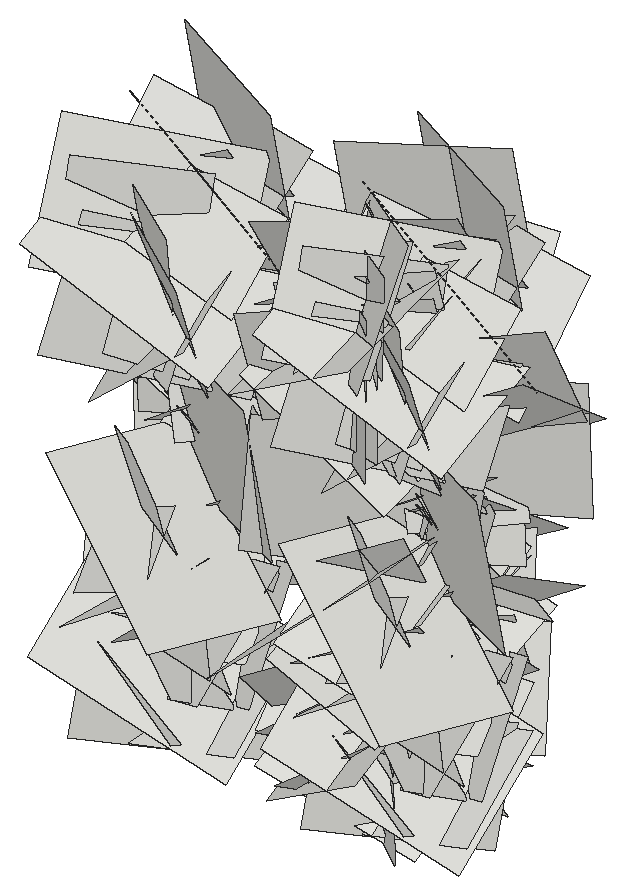
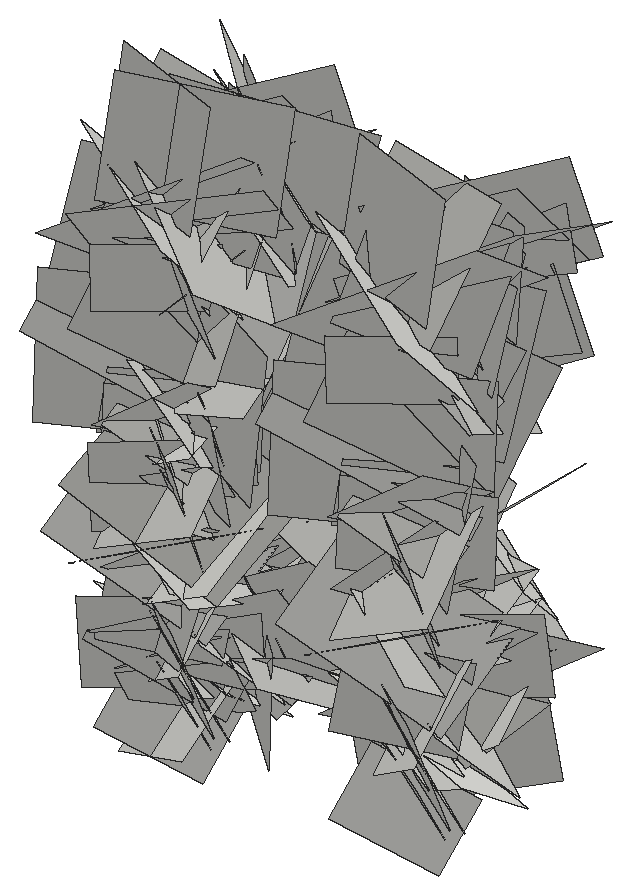
# SketchUp Ruby script. Lengths in inches.
U = 1.inch
M = Sketchup.active_model
def pt(a) = Geom::Point3d.new(a.map { |v| v * U })
def face(e, loops, mat)
  f = e.add_face(loops[0].map { |a| pt(a) })
  loops[1..].each { |l| e.add_face(l.map { |a| pt(a) }).erase! }
  f.material = f.back_material = mat if mat
  f
end
# faces: each face lists its corners as indices into pts; further lists are holes
def faces(e, pts, list, mat = nil) = list.each { |f| face(e, (f[0].is_a?(Array) ? f : [f]).map { |l| l.map { |i| pts[i] } }, mat) }
# xy, xz, yz: faces in a plane at the given z, y or x. An outline is a flat list of corners, or four numbers for a rectangle; further outlines are holes
def ring(l) = l.size == 4 ? [[l[0], l[1]], [l[2], l[1]], [l[2], l[3]], [l[0], l[3]]] : l.each_slice(2).to_a
def flat(e, list, mat, &to3) = list.each { |f| face(e, (f[0].is_a?(Array) ? f : [f]).map { |l| ring(l).map { |u, v| to3.(u, v) } }, mat) }
def xy(e, z, list, mat = nil) = flat(e, list, mat) { |x, y| [x, y, z] }
def xz(e, y, list, mat = nil) = flat(e, list, mat) { |x, z| [x, y, z] }
def yz(e, x, list, mat = nil) = flat(e, list, mat) { |y, z| [x, y, z] }
def lines(e, pts, list) = list.each { |a, b| e.add_line(pt(pts[a]), pt(pts[b])) }
# prism: a flat outline (further loops are holes) pulled along v
def prism(e, loops, v, mat = nil)
  f = face(e, loops, mat); d = Geom::Vector3d.new(v.map { |x| x * U })
  f.pushpull(f.normal.samedirection?(d) ? d.length : -d.length)
end
def box(e, o, s, mat = nil) = prism(e, [[o, [o[0] + s[0], o[1], o[2]], [o[0] + s[0], o[1] + s[1], o[2]], [o[0], o[1] + s[1], o[2]]]], [0, 0, s[2]], mat)
def at(x, y, z, deg = 0) = Geom::Transformation.translation(pt([x, y, z])) * Geom::Transformation.rotation(ORIGIN, Z_AXIS, deg.degrees)
def axes(o, x, y, z) = Geom::Transformation.new([*x, 0, *y, 0, *z, 0, *pt(o).to_a, 1])
def part(name) = M.definitions.add(name)
# library, detail: a bought-in or finely detailed component or shape, given as its bounding box
def library(name, o, s) = part(name).tap { |d| box(d.entities, o, s) }
def detail(e, o, s) = box(e.add_group.entities, o, s)
def put(e, d, t, mat = nil) = e.add_instance(d, t).tap { |i| i.material = mat if mat }
def group(e, t, mat = nil) = e.add_group.tap { |g| g.transformation = t; g.material = mat if mat }.entities
root = M.entities
c1 = part("Component\#6")
p = [[0.01,0,0],[0,3.24,4.54],[4.32,3.24,4.54],[4.33,0,0]]
faces(c1.entities,p,[[0,1,2,3]])
put(root,c1,axes([28.31,207.72,1.15],[0.00392,-0.70388,0.63123],[0.16138,0.62344,0.69431],[-0.98911,0.09893,0.11578]))
put(root,c1,axes([28.31,208.64,6.82],[-0.0498,0.28937,-0.67344],[-0.06797,-0.67386,-0.28508],[-0.77398,0.04056,0.06836]))
put(root,c1,axes([24.34,203.75,8.58],[0.14047,0.70659,0.15459],[-0.00867,0.15861,-0.71798],[0.76665,-0.12767,-0.03644]))
put(root,c1,axes([24.34,201.6875,18.6875],[0.06388,0.10125,0.82658],[-0.05301,0.82768,-0.09774],[0.88113,0.04245,-0.0658]))
put(root,c1,axes([24.34,204.41,7.91],[0.10208,-0.52254,-0.48763],[0.08086,-0.48171,0.53127],[0.75328,0.12252,0.00905]))
put(root,c1,axes([24.34,205.98,8.7],[-0.1184,0.10295,0.88925],[0.12891,0.88959,-0.08771],[0.94011,-0.10902,0.12403]))
put(root,c1,axes([28.31,205.95,7.64],[0.13368,0.21915,0.90835],[0.05222,0.91375,-0.2273],[-0.9891,0.07786,0.11076]))
put(root,c1,axes([28.31,207.38,2.3],[-0.03327,0.56132,-0.40527],[-0.08729,-0.40584,-0.55572],[-0.72866,0.02299,0.08508]))
put(root,c1,axes([24.34,210.56,5.71],[-0.17873,-0.295,-0.9769],[0.02803,-0.99107,0.29472],[1.08133,-0.02307,-0.16911]))
put(root,c1,axes([24.34,206,12.43],[0.16769,0.64159,0.3622],[-0.01184,0.3725,-0.65496],[0.78088,-0.13213,-0.08771]))
put(root,c1,axes([24.34,202.81,3.34],[-0.17899,0.36268,0.93898],[0.06935,0.95405,-0.35673],[1.06473,-0.00117,0.18108]))
put(root,c1,axes([24.34,204.45,21.63],[-0.07523,0.18922,-0.91056],[0.04715,-0.91147,-0.19287],[0.98469,0.0581,-0.06033]))
put(root,c1,axes([28.31,205.65,3.3125],[-0.06993,0.62057,0.27964],[-0.0119,0.27992,-0.62384],[-0.72141,-0.06477,-0.01682]))
put(root,c1,axes([24.34,207.17,17.14],[0.0563,-0.55845,0.63654],[0.00808,0.63808,0.55916],[0.89756,0.02928,-0.04497]))
put(root,c1,axes([28.31,206.6,8.35],[-0.07615,0.29672,0.54367],[-0.07213,0.54022,-0.30383],[-0.65256,-0.09434,-0.02986]))
put(root,c1,axes([28.31,204.05,18.57],[-0.06151,0.80519,-0.14469],[0.18353,-0.12968,-0.7911],[-0.84753,-0.08652,-0.16081]))
put(root,c1,axes([28.31,206.67,12.85],[-0.04142,0.63331,-0.27554],[-0.00251,-0.27611,-0.63426],[-0.73209,-0.03488,0.01776]))
put(root,c1,axes([24.34,205.78,7.5],[-0.02909,0.83454,0.28231],[0.13137,0.2833,-0.8254],[0.92457,-0.01399,0.12617]))
put(root,c1,axes([28.31,206.02,7.14],[-0.00935,0.6115,0.38278],[0.02819,0.38283,-0.61096],[-0.76419,0.00664,-0.02722]))
put(root,c1,axes([28.31,206.15,0.87],[0.01906,0.33732,0.58365],[-0.0637,0.58234,-0.33471],[-0.71172,-0.04309,0.04558]))
put(root,c1,axes([24.34,206.11,11.76],[-0.09648,-0.72051,0.9522],[-0.19874,0.95174,0.70224],[1.25002,0.0957,0.18514]))
put(root,c1,axes([28.31,205.78,22.17],[-0.00372,0.37911,-0.54343],[-0.01311,-0.54338,-0.37899],[-0.70223,0.00813,0.00995]))
put(root,c1,axes([24.34,201.43,15.61],[0.13511,0.17275,0.7909],[0.07376,0.79534,-0.18493],[0.85494,-0.09592,-0.10904]))
put(root,c1,axes([28.31,205.06,0.06],[0.16762,-0.72435,0.3647],[0.00744,0.37278,0.73735],[-0.85961,-0.13802,0.0775]))
put(root,c1,axes([28.31,203.18,8],[-0.06036,-0.35202,0.5516],[0.07606,0.54699,0.35648],[-0.68943,0.09116,-0.00896]))
put(root,c1,axes([24.34,200.34,18.7],[-0.08817,0.51183,1.11442],[-0.20058,1.09825,-0.51853],[1.28435,0.20665,-0.00447]))
put(root,c1,axes([28.31,200.61,7.25],[0.15258,0.77944,0.1154],[0.02035,0.1138,-0.79262],[-0.83497,0.14521,0.00177]))
put(root,c1,axes([28.31,209.54,8.98],[-0.01886,-0.65319,-0.4186],[0.2021,-0.40955,0.63097],[-0.79714,-0.08839,0.16987]))
put(root,c1,axes([28.31,205.68,16.84],[-0.07036,-0.63328,-0.02287],[0.09357,-0.03201,0.6302],[-0.66517,0.06248,0.09107]))
put(root,c1,axes([24.34,211.08,20.1875],[-0.1855,-0.74932,-0.85781],[0.09412,-0.87421,0.74553],[1.20366,-0.04712,-0.19049]))
put(root,c1,axes([24.34,206.49,12.28],[-0.17995,0.92169,-0.62911],[0.1265,-0.6177,-0.93718],[1.17609,0.20746,0.00455]))
put(root,c1,axes([28.31,209.83,18.53],[0.13516,-0.18826,-0.70807],[0.00477,-0.7185,0.19184],[-0.77662,-0.03718,-0.12206]))
put(root,c1,axes([28.31,203.04,6.2],[0.19197,0.78573,-0.28472],[0.09491,-0.3079,-0.79273],[-0.88077,0.13807,-0.14748]))
put(root,c1,axes([28.31,202.62,14.39],[0.09007,0.1944,0.61889],[-0.03503,0.62466,-0.19168],[-0.68673,-0.00637,0.09095]))
put(root,c1,axes([24.34,203.52,7.375],[0.0121,1.00291,-0.55649],[-0.12117,-0.55275,-0.99852],[1.20972,-0.0654,-0.09445]))
put(root,c1,axes([24.34,203.17,19.17],[-0.16233,1.06667,0.75788],[-0.09967,0.75211,-1.07754],[1.38342,0.17935,0.0113]))
put(root,c1,axes([24.34,202.39,0.06],[0.12593,0.12266,1.10922],[-0.15067,1.10807,-0.10731],[1.17331,0.12913,-0.13284]))
put(root,c1,axes([24.34,208.78,4.43],[0.01106,-0.99025,0.53374],[0.00744,0.53381,0.99025],[1.19241,0.00586,-0.01113]))
put(root,c1,axes([24.34,208.53,24.44],[0.00063,0.23668,-1.01361],[0.18606,-0.99912,-0.23319],[1.08753,0.17079,0.04049]))
put(root,c1,axes([24.34,200.25,4.04],[-0.10038,1.14624,0.70824],[-0.13093,0.69961,-1.1488],[1.42222,0.14531,-0.05578]))
put(root,c1,axes([24.34,209.01,4.56],[-0.09462,-0.88739,-0.86898],[0.02241,-0.87218,0.88849],[1.31634,-0.04894,-0.07759]))
put(root,c1,axes([28.31,208.89,13.53],[0.18208,-0.09561,-0.67164],[0.05748,-0.68868,0.1119],[-0.71681,-0.07951,-0.16163]))
put(root,c1,axes([24.34,207.09,15.04],[0.15807,-1.02909,-0.4958],[-0.14338,-0.5124,1.02286],[1.20232,0.07419,0.18716]))
put(root,c1,axes([24.34,204.39,20.61],[0.01972,0.37325,-1.09096],[0.03348,-1.09086,-0.37268],[1.22177,0.02387,0.02782]))
put(root,c1,axes([24.34,203.64,8.5],[0.20575,0.76434,-0.74551],[-0.06488,-0.74852,-0.78336],[1.12991,-0.18216,0.09078]))
put(root,c1,axes([24.34,209.96,4.13],[0.07876,-0.66244,-0.94852],[0.03994,-0.94858,0.66543],[1.2257,0.07348,0.03927]))
put(root,c1,axes([24.34,199.86,19.8],[-0.08167,1.25653,0.46028],[0.00634,0.46136,-1.25848],[1.41846,0.07029,0.03212]))
put(root,c1,axes([24.34,200.79,15.19],[0.21334,0.28139,1.2169],[-0.22593,1.22225,-0.24738],[1.30453,0.16566,-0.24185]))
put(root,c1,axes([24.34,201.07,18.92],[0.13602,0.69446,0.8684],[0.06726,0.86816,-0.70365],[1.17673,-0.1299,-0.06016]))
put(root,c1,axes([24.34,207.71,2.15],[0.07423,-0.90085,-0.6111],[0.34403,-0.56723,0.87337],[1.1014,0.23789,-0.23162]))
put(root,c1,axes([24.34,206.09,10.75],[0.05447,-0.13377,1.26127],[0.13355,1.2566,0.12815],[1.33779,-0.12,-0.06414]))
put(root,c1,axes([24.34,201.2,11.35],[0.2643,1.29708,-0.17492],[-0.19217,-0.14212,-1.31229],[1.37397,-0.26938,-0.1499]))
put(root,c1,axes([24.34,207.28,11.15],[0.07738,-1.09853,0.81062],[0.01823,0.81245,1.09947],[1.44703,0.04851,-0.0572]))
put(root,c1,axes([24.34,205.65,23.04],[0.12198,0.70336,-1.01008],[0.22842,-1.01033,-0.67899],[1.28455,0.11286,0.21665]))
put(root,c1,axes([24.34,205.49,13.28],[0.13832,-0.68419,1.12815],[0.08396,1.13567,0.67959],[1.39605,-0.00051,-0.15265]))
put(root,c1,axes([24.34,206.9375,13.83],[0.19711,0.10382,-1.30915],[0.13395,-1.31749,-0.08653],[1.38559,0.11259,0.1946]))
put(root,c1,axes([38.11,206.9375,13.83],[-0.19711,0.10382,-1.30915],[-0.13395,-1.31749,-0.08653],[-1.38559,0.11259,0.1946]))
put(root,c1,axes([38.11,205.49,13.28],[-0.13832,-0.68419,1.12815],[-0.08396,1.13567,0.67959],[-1.39605,-0.00051,-0.15265]))
put(root,c1,axes([38.11,205.65,23.04],[-0.12198,0.70336,-1.01008],[-0.22842,-1.01033,-0.67899],[-1.28455,0.11286,0.21665]))
put(root,c1,axes([38.11,207.28,11.15],[-0.07738,-1.09853,0.81062],[-0.01823,0.81245,1.09947],[-1.44703,0.04851,-0.0572]))
put(root,c1,axes([38.11,201.2,11.35],[-0.2643,1.29708,-0.17492],[0.19217,-0.14212,-1.31229],[-1.37397,-0.26938,-0.1499]))
put(root,c1,axes([38.11,206.09,10.75],[-0.05447,-0.13377,1.26127],[-0.13355,1.2566,0.12815],[-1.33779,-0.12,-0.06414]))
put(root,c1,axes([38.11,207.71,2.15],[-0.07423,-0.90085,-0.6111],[-0.34403,-0.56723,0.87337],[-1.1014,0.23789,-0.23162]))
put(root,c1,axes([38.11,201.07,18.92],[-0.13602,0.69446,0.8684],[-0.06726,0.86816,-0.70365],[-1.17673,-0.1299,-0.06016]))
put(root,c1,axes([38.11,200.79,15.19],[-0.21334,0.28139,1.2169],[0.22593,1.22225,-0.24738],[-1.30453,0.16566,-0.24185]))
put(root,c1,axes([38.11,199.86,19.8],[0.08167,1.25653,0.46028],[-0.00634,0.46136,-1.25848],[-1.41846,0.07029,0.03212]))
put(root,c1,axes([38.11,209.96,4.13],[-0.07876,-0.66244,-0.94852],[-0.03994,-0.94858,0.66543],[-1.2257,0.07348,0.03927]))
put(root,c1,axes([38.11,203.64,8.5],[-0.20575,0.76434,-0.74551],[0.06488,-0.74852,-0.78336],[-1.12991,-0.18216,0.09078]))
put(root,c1,axes([38.11,204.39,20.61],[-0.01972,0.37325,-1.09096],[-0.03348,-1.09086,-0.37268],[-1.22177,0.02387,0.02782]))
put(root,c1,axes([38.11,207.09,15.04],[-0.15807,-1.02909,-0.4958],[0.14338,-0.5124,1.02286],[-1.20232,0.07419,0.18716]))
put(root,c1,axes([34.14,208.89,13.53],[-0.18208,-0.09561,-0.67164],[-0.05748,-0.68868,0.1119],[0.71681,-0.07951,-0.16163]))
put(root,c1,axes([38.11,209.01,4.56],[0.09462,-0.88739,-0.86898],[-0.02241,-0.87218,0.88849],[-1.31634,-0.04894,-0.07759]))
put(root,c1,axes([38.11,200.25,4.04],[0.10038,1.14624,0.70824],[0.13093,0.69961,-1.1488],[-1.42222,0.14531,-0.05578]))
put(root,c1,axes([38.11,208.53,24.44],[-0.00063,0.23668,-1.01361],[-0.18606,-0.99912,-0.23319],[-1.08753,0.17079,0.04049]))
put(root,c1,axes([38.11,208.78,4.43],[-0.01106,-0.99025,0.53374],[-0.00744,0.53381,0.99025],[-1.19241,0.00586,-0.01113]))
put(root,c1,axes([38.11,202.39,0.06],[-0.12593,0.12266,1.10922],[0.15067,1.10807,-0.10731],[-1.17331,0.12913,-0.13284]))
put(root,c1,axes([38.11,203.17,19.17],[0.16233,1.06667,0.75788],[0.09967,0.75211,-1.07754],[-1.38342,0.17935,0.0113]))
put(root,c1,axes([38.11,203.52,7.375],[-0.0121,1.00291,-0.55649],[0.12117,-0.55275,-0.99852],[-1.20972,-0.0654,-0.09445]))
put(root,c1,axes([34.14,202.62,14.39],[-0.09007,0.1944,0.61889],[0.03503,0.62466,-0.19168],[0.68673,-0.00637,0.09095]))
put(root,c1,axes([34.14,203.04,6.2],[-0.19197,0.78573,-0.28472],[-0.09491,-0.3079,-0.79273],[0.88077,0.13807,-0.14748]))
put(root,c1,axes([34.14,209.83,18.53],[-0.13516,-0.18826,-0.70807],[-0.00477,-0.7185,0.19184],[0.77662,-0.03718,-0.12206]))
put(root,c1,axes([38.11,206.49,12.28],[0.17995,0.92169,-0.62911],[-0.1265,-0.6177,-0.93718],[-1.17609,0.20746,0.00455]))
put(root,c1,axes([38.11,211.08,20.1875],[0.1855,-0.74932,-0.85781],[-0.09412,-0.87421,0.74553],[-1.20366,-0.04712,-0.19049]))
put(root,c1,axes([34.14,205.68,16.84],[0.07036,-0.63328,-0.02287],[-0.09357,-0.03201,0.6302],[0.66517,0.06248,0.09107]))
put(root,c1,axes([34.14,209.54,8.98],[0.01886,-0.65319,-0.4186],[-0.2021,-0.40955,0.63097],[0.79714,-0.08839,0.16987]))
put(root,c1,axes([34.14,200.61,7.25],[-0.15258,0.77944,0.1154],[-0.02035,0.1138,-0.79262],[0.83497,0.14521,0.00177]))
put(root,c1,axes([38.11,200.34,18.7],[0.08817,0.51183,1.11442],[0.20058,1.09825,-0.51853],[-1.28435,0.20665,-0.00447]))
put(root,c1,axes([34.14,203.18,8],[0.06036,-0.35202,0.5516],[-0.07606,0.54699,0.35648],[0.68943,0.09116,-0.00896]))
put(root,c1,axes([34.14,205.06,0.06],[-0.16762,-0.72435,0.3647],[-0.00744,0.37278,0.73735],[0.85961,-0.13802,0.0775]))
put(root,c1,axes([38.11,201.43,15.61],[-0.13511,0.17275,0.7909],[-0.07376,0.79534,-0.18493],[-0.85494,-0.09592,-0.10904]))
put(root,c1,axes([34.14,205.78,22.17],[0.00372,0.37911,-0.54343],[0.01311,-0.54338,-0.37899],[0.70223,0.00813,0.00995]))
put(root,c1,axes([38.11,206.11,11.76],[0.09648,-0.72051,0.9522],[0.19874,0.95174,0.70224],[-1.25002,0.0957,0.18514]))
put(root,c1,axes([34.14,206.15,0.87],[-0.01906,0.33732,0.58365],[0.0637,0.58234,-0.33471],[0.71172,-0.04309,0.04558]))
put(root,c1,axes([34.14,206.02,7.14],[0.00935,0.6115,0.38278],[-0.02819,0.38283,-0.61096],[0.76419,0.00664,-0.02722]))
put(root,c1,axes([38.11,205.78,7.5],[0.02909,0.83454,0.28231],[-0.13137,0.2833,-0.8254],[-0.92457,-0.01399,0.12617]))
put(root,c1,axes([34.14,206.67,12.85],[0.04142,0.63331,-0.27554],[0.00251,-0.27611,-0.63426],[0.73209,-0.03488,0.01776]))
put(root,c1,axes([34.14,204.05,18.57],[0.06151,0.80519,-0.14469],[-0.18353,-0.12968,-0.7911],[0.84753,-0.08652,-0.16081]))
put(root,c1,axes([34.14,206.6,8.35],[0.07615,0.29672,0.54367],[0.07213,0.54022,-0.30383],[0.65256,-0.09434,-0.02986]))
put(root,c1,axes([38.11,207.17,17.14],[-0.0563,-0.55845,0.63654],[-0.00808,0.63808,0.55916],[-0.89756,0.02928,-0.04497]))
put(root,c1,axes([34.14,205.65,3.3125],[0.06993,0.62057,0.27964],[0.0119,0.27992,-0.62384],[0.72141,-0.06477,-0.01682]))
put(root,c1,axes([38.11,204.45,21.63],[0.07523,0.18922,-0.91056],[-0.04715,-0.91147,-0.19287],[-0.98469,0.0581,-0.06033]))
put(root,c1,axes([38.11,202.81,3.34],[0.17899,0.36268,0.93898],[-0.06935,0.95405,-0.35673],[-1.06473,-0.00117,0.18108]))
put(root,c1,axes([38.11,206,12.43],[-0.16769,0.64159,0.3622],[0.01184,0.3725,-0.65496],[-0.78088,-0.13213,-0.08771]))
put(root,c1,axes([38.11,210.56,5.71],[0.17873,-0.295,-0.9769],[-0.02803,-0.99107,0.29472],[-1.08133,-0.02307,-0.16911]))
put(root,c1,axes([34.14,207.38,2.3],[0.03327,0.56132,-0.40527],[0.08729,-0.40584,-0.55572],[0.72866,0.02299,0.08508]))
put(root,c1,axes([34.14,205.95,7.64],[-0.13368,0.21915,0.90835],[-0.05222,0.91375,-0.2273],[0.9891,0.07786,0.11076]))
put(root,c1,axes([38.11,205.98,8.7],[0.1184,0.10295,0.88925],[-0.12891,0.88959,-0.08771],[-0.94011,-0.10902,0.12403]))
put(root,c1,axes([38.11,204.41,7.91],[-0.10208,-0.52254,-0.48763],[-0.08086,-0.48171,0.53127],[-0.75328,0.12252,0.00905]))
put(root,c1,axes([38.11,201.6875,18.6875],[-0.06388,0.10125,0.82658],[0.05301,0.82768,-0.09774],[-0.88113,0.04245,-0.0658]))
put(root,c1,axes([38.11,203.75,8.58],[-0.14047,0.70659,0.15459],[0.00867,0.15861,-0.71798],[-0.76665,-0.12767,-0.03644]))
put(root,c1,axes([34.14,208.64,6.82],[0.0498,0.28937,-0.67344],[0.06797,-0.67386,-0.28508],[0.77398,0.04056,0.06836]))
put(root,c1,axes([34.14,207.72,1.15],[-0.00392,-0.70388,0.63123],[-0.16138,0.62344,0.69431],[0.98911,0.09893,0.11578]))
put(root,c1,axes([38.11,207.72,1.15],[0.00392,-0.70388,0.63123],[0.16138,0.62344,0.69431],[-0.98911,0.09893,0.11578]))
put(root,c1,axes([38.11,208.64,6.82],[-0.0498,0.28937,-0.67344],[-0.06797,-0.67386,-0.28508],[-0.77398,0.04056,0.06836]))
put(root,c1,axes([34.14,203.75,8.58],[0.14047,0.70659,0.15459],[-0.00867,0.15861,-0.71798],[0.76665,-0.12767,-0.03644]))
put(root,c1,axes([34.14,201.6875,18.6875],[0.06388,0.10125,0.82658],[-0.05301,0.82768,-0.09774],[0.88113,0.04245,-0.0658]))
put(root,c1,axes([34.14,204.41,7.91],[0.10208,-0.52254,-0.48763],[0.08086,-0.48171,0.53127],[0.75328,0.12252,0.00905]))
put(root,c1,axes([34.14,205.98,8.7],[-0.1184,0.10295,0.88925],[0.12891,0.88959,-0.08771],[0.94011,-0.10902,0.12403]))
put(root,c1,axes([38.11,205.95,7.64],[0.13368,0.21915,0.90835],[0.05222,0.91375,-0.2273],[-0.9891,0.07786,0.11076]))
put(root,c1,axes([38.11,207.38,2.3],[-0.03327,0.56132,-0.40527],[-0.08729,-0.40584,-0.55572],[-0.72866,0.02299,0.08508]))
put(root,c1,axes([34.14,210.56,5.71],[-0.17873,-0.295,-0.9769],[0.02803,-0.99107,0.29472],[1.08133,-0.02307,-0.16911]))
put(root,c1,axes([34.14,206,12.43],[0.16769,0.64159,0.3622],[-0.01184,0.3725,-0.65496],[0.78088,-0.13213,-0.08771]))
put(root,c1,axes([34.14,202.81,3.34],[-0.17899,0.36268,0.93898],[0.06935,0.95405,-0.35673],[1.06473,-0.00117,0.18108]))
put(root,c1,axes([34.14,204.45,21.63],[-0.07523,0.18922,-0.91056],[0.04715,-0.91147,-0.19287],[0.98469,0.0581,-0.06033]))
put(root,c1,axes([38.11,205.65,3.3125],[-0.06993,0.62057,0.27964],[-0.0119,0.27992,-0.62384],[-0.72141,-0.06477,-0.01682]))
put(root,c1,axes([34.14,207.17,17.14],[0.0563,-0.55845,0.63654],[0.00808,0.63808,0.55916],[0.89756,0.02928,-0.04497]))
put(root,c1,axes([38.11,206.6,8.35],[-0.07615,0.29672,0.54367],[-0.07213,0.54022,-0.30383],[-0.65256,-0.09434,-0.02986]))
put(root,c1,axes([38.11,204.05,18.57],[-0.06151,0.80519,-0.14469],[0.18353,-0.12968,-0.7911],[-0.84753,-0.08652,-0.16081]))
put(root,c1,axes([38.11,206.67,12.85],[-0.04142,0.63331,-0.27554],[-0.00251,-0.27611,-0.63426],[-0.73209,-0.03488,0.01776]))
put(root,c1,axes([34.14,205.78,7.5],[-0.02909,0.83454,0.28231],[0.13137,0.2833,-0.8254],[0.92457,-0.01399,0.12617]))
put(root,c1,axes([38.11,206.02,7.14],[-0.00935,0.6115,0.38278],[0.02819,0.38283,-0.61096],[-0.76419,0.00664,-0.02722]))
put(root,c1,axes([38.11,206.15,0.87],[0.01906,0.33732,0.58365],[-0.0637,0.58234,-0.33471],[-0.71172,-0.04309,0.04558]))
put(root,c1,axes([34.14,206.11,11.76],[-0.09648,-0.72051,0.9522],[-0.19874,0.95174,0.70224],[1.25002,0.0957,0.18514]))
put(root,c1,axes([38.11,205.78,22.17],[-0.00372,0.37911,-0.54343],[-0.01311,-0.54338,-0.37899],[-0.70223,0.00813,0.00995]))
put(root,c1,axes([34.14,201.43,15.61],[0.13511,0.17275,0.7909],[0.07376,0.79534,-0.18493],[0.85494,-0.09592,-0.10904]))
put(root,c1,axes([38.11,205.06,0.06],[0.16762,-0.72435,0.3647],[0.00744,0.37278,0.73735],[-0.85961,-0.13802,0.0775]))
put(root,c1,axes([38.11,203.18,8],[-0.06036,-0.35202,0.5516],[0.07606,0.54699,0.35648],[-0.68943,0.09116,-0.00896]))
put(root,c1,axes([34.14,200.34,18.7],[-0.08817,0.51183,1.11442],[-0.20058,1.09825,-0.51853],[1.28435,0.20665,-0.00447]))
put(root,c1,axes([38.11,200.61,7.25],[0.15258,0.77944,0.1154],[0.02035,0.1138,-0.79262],[-0.83497,0.14521,0.00177]))
put(root,c1,axes([38.11,209.54,8.98],[-0.01886,-0.65319,-0.4186],[0.2021,-0.40955,0.63097],[-0.79714,-0.08839,0.16987]))
put(root,c1,axes([38.11,205.68,16.84],[-0.07036,-0.63328,-0.02287],[0.09357,-0.03201,0.6302],[-0.66517,0.06248,0.09107]))
put(root,c1,axes([34.14,211.08,20.1875],[-0.1855,-0.74932,-0.85781],[0.09412,-0.87421,0.74553],[1.20366,-0.04712,-0.19049]))
put(root,c1,axes([34.14,206.49,12.28],[-0.17995,0.92169,-0.62911],[0.1265,-0.6177,-0.93718],[1.17609,0.20746,0.00455]))
put(root,c1,axes([38.11,209.83,18.53],[0.13516,-0.18826,-0.70807],[0.00477,-0.7185,0.19184],[-0.77662,-0.03718,-0.12206]))
put(root,c1,axes([38.11,203.04,6.2],[0.19197,0.78573,-0.28472],[0.09491,-0.3079,-0.79273],[-0.88077,0.13807,-0.14748]))
put(root,c1,axes([38.11,202.62,14.39],[0.09007,0.1944,0.61889],[-0.03503,0.62466,-0.19168],[-0.68673,-0.00637,0.09095]))
put(root,c1,axes([34.14,203.52,7.375],[0.0121,1.00291,-0.55649],[-0.12117,-0.55275,-0.99852],[1.20972,-0.0654,-0.09445]))
put(root,c1,axes([34.14,203.17,19.17],[-0.16233,1.06667,0.75788],[-0.09967,0.75211,-1.07754],[1.38342,0.17935,0.0113]))
put(root,c1,axes([34.14,202.39,0.06],[0.12593,0.12266,1.10922],[-0.15067,1.10807,-0.10731],[1.17331,0.12913,-0.13284]))
put(root,c1,axes([34.14,208.78,4.43],[0.01106,-0.99025,0.53374],[0.00744,0.53381,0.99025],[1.19241,0.00586,-0.01113]))
put(root,c1,axes([34.14,208.53,24.44],[0.00063,0.23668,-1.01361],[0.18606,-0.99912,-0.23319],[1.08753,0.17079,0.04049]))
put(root,c1,axes([34.14,200.25,4.04],[-0.10038,1.14624,0.70824],[-0.13093,0.69961,-1.1488],[1.42222,0.14531,-0.05578]))
put(root,c1,axes([34.14,209.01,4.56],[-0.09462,-0.88739,-0.86898],[0.02241,-0.87218,0.88849],[1.31634,-0.04894,-0.07759]))
put(root,c1,axes([38.11,208.89,13.53],[0.18208,-0.09561,-0.67164],[0.05748,-0.68868,0.1119],[-0.71681,-0.07951,-0.16163]))
put(root,c1,axes([34.14,207.09,15.04],[0.15807,-1.02909,-0.4958],[-0.14338,-0.5124,1.02286],[1.20232,0.07419,0.18716]))
put(root,c1,axes([34.14,204.39,20.61],[0.01972,0.37325,-1.09096],[0.03348,-1.09086,-0.37268],[1.22177,0.02387,0.02782]))
put(root,c1,axes([34.14,203.64,8.5],[0.20575,0.76434,-0.74551],[-0.06488,-0.74852,-0.78336],[1.12991,-0.18216,0.09078]))
put(root,c1,axes([34.14,209.96,4.13],[0.07876,-0.66244,-0.94852],[0.03994,-0.94858,0.66543],[1.2257,0.07348,0.03927]))
put(root,c1,axes([34.14,199.86,19.8],[-0.08167,1.25653,0.46028],[0.00634,0.46136,-1.25848],[1.41846,0.07029,0.03212]))
put(root,c1,axes([34.14,200.79,15.19],[0.21334,0.28139,1.2169],[-0.22593,1.22225,-0.24738],[1.30453,0.16566,-0.24185]))
put(root,c1,axes([34.14,201.07,18.92],[0.13602,0.69446,0.8684],[0.06726,0.86816,-0.70365],[1.17673,-0.1299,-0.06016]))
put(root,c1,axes([34.14,207.71,2.15],[0.07423,-0.90085,-0.6111],[0.34403,-0.56723,0.87337],[1.1014,0.23789,-0.23162]))
put(root,c1,axes([34.14,206.09,10.75],[0.05447,-0.13377,1.26127],[0.13355,1.2566,0.12815],[1.33779,-0.12,-0.06414]))
put(root,c1,axes([34.14,201.2,11.35],[0.2643,1.29708,-0.17492],[-0.19217,-0.14212,-1.31229],[1.37397,-0.26938,-0.1499]))
put(root,c1,axes([34.14,207.28,11.15],[0.07738,-1.09853,0.81062],[0.01823,0.81245,1.09947],[1.44703,0.04851,-0.0572]))
put(root,c1,axes([34.14,205.65,23.04],[0.12198,0.70336,-1.01008],[0.22842,-1.01033,-0.67899],[1.28455,0.11286,0.21665]))
put(root,c1,axes([34.14,205.49,13.28],[0.13832,-0.68419,1.12815],[0.08396,1.13567,0.67959],[1.39605,-0.00051,-0.15265]))
put(root,c1,axes([34.14,206.9375,13.83],[0.19711,0.10382,-1.30915],[0.13395,-1.31749,-0.08653],[1.38559,0.11259,0.1946]))
